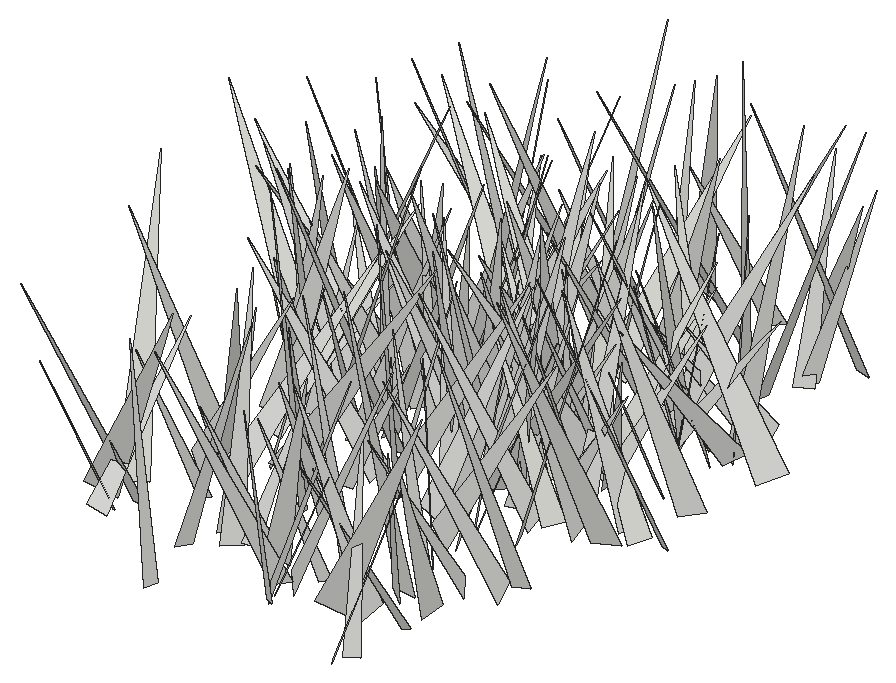
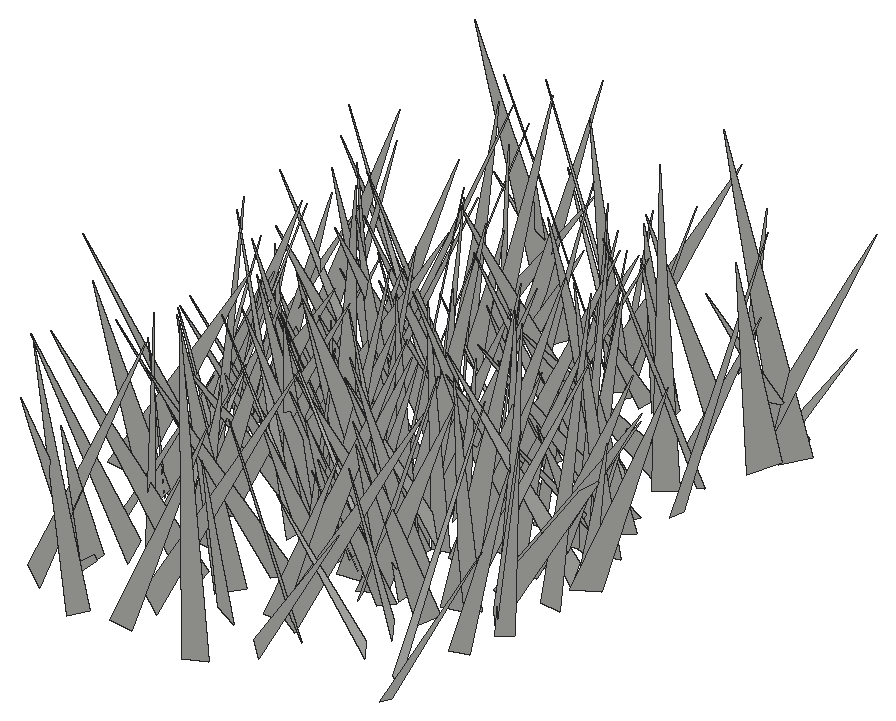
# SketchUp Ruby script. Lengths in inches.
U = 1.inch
M = Sketchup.active_model
def pt(a) = Geom::Point3d.new(a.map { |v| v * U })
def face(e, loops, mat)
  f = e.add_face(loops[0].map { |a| pt(a) })
  loops[1..].each { |l| e.add_face(l.map { |a| pt(a) }).erase! }
  f.material = f.back_material = mat if mat
  f
end
# faces: each face lists its corners as indices into pts; further lists are holes
def faces(e, pts, list, mat = nil) = list.each { |f| face(e, (f[0].is_a?(Array) ? f : [f]).map { |l| l.map { |i| pts[i] } }, mat) }
# xy, xz, yz: faces in a plane at the given z, y or x. An outline is a flat list of corners, or four numbers for a rectangle; further outlines are holes
def ring(l) = l.size == 4 ? [[l[0], l[1]], [l[2], l[1]], [l[2], l[3]], [l[0], l[3]]] : l.each_slice(2).to_a
def flat(e, list, mat, &to3) = list.each { |f| face(e, (f[0].is_a?(Array) ? f : [f]).map { |l| ring(l).map { |u, v| to3.(u, v) } }, mat) }
def xy(e, z, list, mat = nil) = flat(e, list, mat) { |x, y| [x, y, z] }
def xz(e, y, list, mat = nil) = flat(e, list, mat) { |x, z| [x, y, z] }
def yz(e, x, list, mat = nil) = flat(e, list, mat) { |y, z| [x, y, z] }
def lines(e, pts, list) = list.each { |a, b| e.add_line(pt(pts[a]), pt(pts[b])) }
# prism: a flat outline (further loops are holes) pulled along v
def prism(e, loops, v, mat = nil)
  f = face(e, loops, mat); d = Geom::Vector3d.new(v.map { |x| x * U })
  f.pushpull(f.normal.samedirection?(d) ? d.length : -d.length)
end
def box(e, o, s, mat = nil) = prism(e, [[o, [o[0] + s[0], o[1], o[2]], [o[0] + s[0], o[1] + s[1], o[2]], [o[0], o[1] + s[1], o[2]]]], [0, 0, s[2]], mat)
def at(x, y, z, deg = 0) = Geom::Transformation.translation(pt([x, y, z])) * Geom::Transformation.rotation(ORIGIN, Z_AXIS, deg.degrees)
def axes(o, x, y, z) = Geom::Transformation.new([*x, 0, *y, 0, *z, 0, *pt(o).to_a, 1])
def part(name) = M.definitions.add(name)
# library, detail: a bought-in or finely detailed component or shape, given as its bounding box
def library(name, o, s) = part(name).tap { |d| box(d.entities, o, s) }
def detail(e, o, s) = box(e.add_group.entities, o, s)
def put(e, d, t, mat = nil) = e.add_instance(d, t).tap { |i| i.material = mat if mat }
def group(e, t, mat = nil) = e.add_group.tap { |g| g.transformation = t; g.material = mat if mat }.entities
root = M.entities
c1 = part("fur_instance\#9")
p = [[0.8125,0,1.79],[0.67,-0.02,1.48],[0,-0.11,0],[0,0.11,0]]
faces(c1.entities,p,[[0,1,2,3]])
put(root,c1,axes([454.45,190.55,-21.66],[-5.80896,4.38047,0.69826],[4.41604,5.60261,1.59041],[-0.41794,-1.68592,7.09952]))
put(root,c1,axes([455.25,204.84,-21.66],[-4.70731,-0.314,0.0439],[-0.28456,4.4722,1.47573],[0.13983,-1.46975,4.48103]))
put(root,c1,axes([455.15,189.58,-21.66],[0.45308,4.94253,1.25959],[4.74966,-0.86975,1.70432],[-1.859,-1.01755,4.66145]))
put(root,c1,axes([455.2,175.94,-21.66],[-6.50457,4.89284,0.5628],[4.72218,6.46057,-1.59001],[1.39918,0.94188,7.98255]))
put(root,c1,axes([456.21,173.26,-21.66],[-2.80536,-2.90649,0.0794],[-2.63209,2.49174,-1.78533],[-1.23535,1.29136,3.62358]))
put(root,c1,axes([457.82,191.1875,-21.66],[-5.05806,4.73106,0.08976],[4.36112,4.60989,2.7757],[-1.83619,-2.08349,6.34527]))
put(root,c1,axes([456.97,193.71,-21.66],[-0.73144,-5.99959,0.26703],[-5.39662,0.53861,-2.681],[-2.63493,0.56233,5.41685]))
put(root,c1,axes([456.87,174.45,-21.66],[-2.83632,-6.0499,0.28173],[-5.90232,2.69141,-1.62612],[-1.35766,0.93829,6.48088]))
put(root,c1,axes([456.02,195.5,-21.66],[-4.69579,-3.74143,2.09942],[-4.25802,4.44495,-1.60248],[0.52452,2.58851,5.78625]))
put(root,c1,axes([455.65,182.05,-21.66],[-7.05336,-2.15617,1.71578],[-1.62887,7.06566,2.18314],[2.22256,-1.66441,7.04506]))
put(root,c1,axes([457.25,190.05,-21.66],[-3.27496,5.22829,1.96451],[5.47571,2.5569,2.32348],[-1.10043,-2.83671,5.71505]))
put(root,c1,axes([455.375,199.04,-21.66],[3.46395,-3.11936,0.86631],[-2.7787,-3.51575,-1.54862],[-1.66124,-0.62369,4.39672]))
put(root,c1,axes([454.77,192.86,-21.66],[-2.27672,-7.40144,1.23154],[-7.29478,2.48469,1.44709],[1.75622,0.72557,7.60728]))
put(root,c1,axes([456.03,203.05,-21.66],[-4.76858,-5.56642,0.65425],[-5.40433,4.79429,1.40014],[1.48534,-0.42682,7.19472]))
put(root,c1,axes([459.25,193.09,-21.66],[-5.59942,-5.49473,0.70955],[-5.42162,5.22657,-2.3104],[-1.14084,2.13071,7.49717]))
put(root,c1,axes([455.63,172.7,-21.66],[-0.63862,5.35473,0.03552],[5.1577,0.62471,-1.44573],[1.43964,0.13724,5.19527]))
put(root,c1,axes([458.1,185.21,-21.66],[-3.16034,-1.96863,0.75138],[-2.10046,2.8354,-1.40585],[-0.16774,1.5852,3.44773]))
put(root,c1,axes([454.72,196.38,-21.66],[-1.50636,-7.45489,0.25307],[-6.77182,1.47502,3.14252],[3.12761,-0.39686,6.92598]))
put(root,c1,axes([455.55,187.31,-21.66],[-0.42435,-6.57592,2.54627],[-6.78158,1.0798,1.65847],[1.93298,2.34469,6.37748]))
put(root,c1,axes([457.88,186.42,-21.66],[-4.70225,1.57903,0.9136],[0.9953,4.33742,-2.37389],[1.52885,2.03289,4.35536]))
put(root,c1,axes([458.82,176.93,-21.66],[-0.44719,-4.16584,0.88919],[-4.01944,0.11666,-1.47491],[-1.41032,0.98845,3.92158]))
put(root,c1,axes([459.29,189.81,-21.66],[-1.35626,4.67986,0.4324],[4.48876,1.15652,1.56235],[-1.3925,-0.82998,4.61514]))
put(root,c1,axes([455.82,189.625,-21.66],[6.85876,3.23862,0.41321],[3.02392,-6.66397,2.03701],[-1.23097,1.67477,7.30628]))
put(root,c1,axes([457.08,187.68,-21.66],[-3.46246,-6.72611,1.90114],[-6.59046,3.84836,1.61233],[2.32826,0.89059,7.39118]))
put(root,c1,axes([457.16,187.43,-21.66],[4.65411,-4.15615,0.09318],[-4.0063,-4.52139,-1.56511],[-1.10988,-1.10744,6.04026]))
put(root,c1,axes([456.25,186.42,-21.66],[-0.23722,4.19444,0.05409],[3.55446,0.22976,-2.22834],[2.22756,0.08005,3.56147]))
put(root,c1,axes([454.51,174.41,-21.66],[3.10816,-7.62871,0.22312],[-7.12075,-2.81203,3.04879],[2.74626,1.34273,7.65263]))
put(root,c1,axes([461.44,190.13,-21.66],[0.20171,6.63601,2.13173],[6.14884,-1.17367,3.07178],[-3.28217,-1.79094,5.8857]))
put(root,c1,axes([456.18,187.3125,-21.66],[3.26284,4.45559,0.15103],[4.26787,-3.06768,-1.7017],[1.28856,-1.1217,5.25381]))
put(root,c1,axes([459.2,199.33,-21.66],[4.53649,3.63122,1.57008],[3.09166,-4.74451,2.04009],[-2.46831,0.73111,5.44092]))
put(root,c1,axes([456.54,185.21,-21.66],[0.11593,7.32982,3.76994],[7.80213,1.11829,-2.4142],[2.6581,-3.60212,6.9218]))
put(root,c1,axes([460.31,190.17,-21.66],[2.04194,-5.37013,1.21962],[-4.97283,-2.35693,-2.05211],[-2.36574,0.31918,5.36625]))
put(root,c1,axes([457.5,195.51,-21.66],[0.9975,-5.62203,0.93729],[-5.55991,-0.75041,1.41599],[1.25425,1.14473,5.53148]))
put(root,c1,axes([457.11,183.9375,-21.66],[-1.44675,6.62808,0.1342],[5.91861,1.35324,-3.03008],[2.98656,0.529,6.06986]))
put(root,c1,axes([462.35,197.03,-21.66],[-5.71185,4.45959,0.23835],[4.39877,5.55102,1.55146],[-0.77178,-1.36683,7.07857]))
put(root,c1,axes([459.51,181.11,-21.66],[3.36886,3.17868,0.5186],[2.75759,-3.23451,1.91201],[-1.66392,1.0752,4.2187]))
put(root,c1,axes([458.05,195.9,-21.66],[7.18044,-3.7228,0.21814],[-3.29243,-6.55088,-3.42221],[-1.75122,-2.94828,7.32847]))
put(root,c1,axes([460.53,192.27,-21.66],[0.98136,-7.62341,0.77855],[-7.49654,-1.11781,-1.49599],[-1.58884,0.56543,7.53933]))
put(root,c1,axes([456.37,179.33,-21.66],[3.98085,5.13777,1.04709],[4.9615,-3.26572,-2.83883],[1.69606,-2.50573,5.84679]))
put(root,c1,axes([462.77,197.01,-21.66],[-7.75285,-2.01113,0.68817],[-2.11722,7.53738,-1.82488],[0.1887,1.94117,7.79879]))
put(root,c1,axes([461.73,187.27,-21.66],[2.76553,6.92914,2.18566],[6.51494,-3.40021,2.53621],[-3.21647,-0.92942,7.01632]))
put(root,c1,axes([459.09,201.59,-21.66],[4.51704,3.2359,0.24642],[3.07452,-4.40221,1.45028],[-1.0388,1.04161,5.3639]))
put(root,c1,axes([457.54,180.54,-21.66],[7.63705,-2.12328,0.08153],[-2.0044,-7.29978,-2.35267],[-0.70524,-2.24596,7.56953]))
put(root,c1,axes([458.59,179.22,-21.66],[-3.50989,5.55769,0.51718],[4.45011,3.15505,-3.70364],[3.36927,1.62248,5.4305]))
put(root,c1,axes([458.46,197.51,-21.66],[4.54931,-2.96003,1.24819],[-3.21199,-4.22741,1.68171],[-0.05363,2.09362,5.16041]))
put(root,c1,axes([462.23,168.58,-21.66],[-5.98582,-0.44068,0.88109],[-0.67667,5.78235,-1.70504],[0.71598,1.78068,5.75475]))
put(root,c1,axes([463.15,204.84,-21.66],[-3.16767,-3.69393,0.44061],[-3.42422,2.66901,-2.24153],[-1.45395,1.76199,4.31912]))
put(root,c1,axes([463.41,186.07,-21.66],[-3.74944,-6.99723,1.04952],[-6.92154,3.38084,-2.18706],[-1.468,1.93125,7.63127]))
put(root,c1,axes([460.03,187.05,-21.66],[-1.799,-4.93024,0.4482],[-4.7112,1.85147,1.45641],[1.52075,-0.09654,5.04207]))
put(root,c1,axes([463.42,178.71,-21.66],[-7.24108,-2.76695,1.69952],[-3.23599,6.49389,-3.21487],[0.2698,3.62643,7.05364]))
put(root,c1,axes([463.7,201.8,-21.66],[-2.5504,-6.61055,0.06946],[-6.29815,2.40698,-2.17909],[-2.00934,0.84606,6.74207]))
put(root,c1,axes([460.77,194.97,-21.66],[7.1916,2.06862,2.54607],[1.20326,-7.37063,2.58975],[-3.05186,1.96861,7.0208]))
put(root,c1,axes([463.9,183.93,-21.66],[-7.08449,-0.21202,0.14595],[-0.16992,6.87165,1.73429],[0.19334,-1.72965,6.8722]))
put(root,c1,axes([461.72,174.9,-21.66],[4.93577,0.48548,2.66433],[-0.37318,-5.36398,1.66873],[-2.68236,1.63958,4.67042]))
put(root,c1,axes([461.125,185.51,-21.66],[-5.44791,2.04028,1.98238],[0.64646,5.0587,-3.42987],[2.77031,2.83181,4.69878]))
put(root,c1,axes([462.83,174.07,-21.66],[-6.34351,2.24327,1.15963],[1.89857,6.30395,-1.80908],[1.66506,1.35834,6.48071]))
put(root,c1,axes([461.02,172.59,-21.66],[5.70541,0.17051,1.69377],[-0.31532,-5.71566,1.63753],[-1.67287,1.65887,5.46803]))
put(root,c1,axes([462.67,195.15,-21.66],[-4.26385,3.34064,0.29483],[3.15748,4.15963,-1.468],[1.13011,0.98225,5.21395]))
put(root,c1,axes([463.83,188.33,-21.66],[-6.21207,0.31771,0.7174],[0.09871,5.99609,-1.80072],[0.77837,1.77522,5.95384]))
put(root,c1,axes([461.47,182.03,-21.66],[6.96857,3.90701,1.2479],[3.36407,-6.85211,2.66731],[-2.34628,1.77954,7.53068]))
put(root,c1,axes([464.39,189.52,-21.66],[-6.62778,2.24684,1.33683],[2.5489,6.36376,1.94128],[0.58185,-2.2841,6.72363]))
put(root,c1,axes([464.28,201.01,-21.66],[-0.7633,-7.78268,1.04828],[-7.63293,0.4877,-1.93706],[-1.84592,1.20152,7.57632]))
put(root,c1,axes([462.75,202.24,-21.66],[4.10406,6.33899,0.98584],[6.11766,-4.2195,1.66374],[-1.93105,0.10466,7.36601]))
put(root,c1,axes([460.75,196.53,-21.66],[6.83601,2.20523,1.02382],[2.40175,-6.59991,-1.82073],[-0.37792,-2.05437,6.94831]))
put(root,c1,axes([462.09,180.84,-21.66],[5.97611,0.87511,2.00016],[1.66713,-5.59279,-2.53411],[-1.40966,-2.90435,5.48252]))
put(root,c1,axes([462.76,191.13,-21.66],[5.4592,3.52611,0.65952],[3.05756,-5.20187,2.50265],[-1.87611,1.78282,5.99776]))
put(root,c1,axes([462.05,187.125,-21.66],[6.79493,0.95964,1.40947],[0.56386,-6.72962,1.86359],[-1.60922,1.6941,6.60447]))
put(root,c1,axes([460.98,197.55,-21.66],[0.71966,5.69009,1.64056],[5.43341,0.02279,-2.46251],[2.35511,-1.79132,5.17987]))
put(root,c1,axes([464.45,201.9,-21.66],[1.33499,-4.14938,1.03511],[-3.92508,-1.61935,-1.42916],[-1.69781,0.48101,4.1179]))
put(root,c1,axes([462.26,191.83,-21.66],[-0.76172,-5.93829,1.58025],[-5.83151,1.20063,1.7008],[1.93753,1.27903,5.74028]))
put(root,c1,axes([463.48,174.57,-21.66],[-2.96386,2.60362,0.59977],[2.15648,2.85999,-1.75873],[1.5774,0.98217,3.53132]))
put(root,c1,axes([466.95,194.54,-21.66],[-5.54363,5.04114,0.10568],[4.92423,5.3789,1.72499],[-1.08457,-1.34553,7.29173]))
put(root,c1,axes([465.28,189.49,-21.66],[1.50286,-5.49819,1.33251],[-5.18917,-1.88889,-1.94134],[-2.25347,0.68284,5.35909]))
put(root,c1,axes([466.13,182.54,-21.66],[-6.09623,-2.24198,1.5344],[-2.70516,5.35755,-2.91953],[0.25098,3.28863,5.80232]))
put(root,c1,axes([464.22,195.45,-21.66],[-4.08665,1.67614,0.95166],[1.15635,3.91687,-1.93308],[1.54207,1.50482,3.97156]))
put(root,c1,axes([463.8,192.24,-21.66],[5.79186,-5.56058,1.06137],[-5.14067,-5.80215,-2.34538],[-2.37068,-1.00358,7.67886]))
put(root,c1,axes([464.62,174.78,-21.66],[-4.80536,-1.45342,1.08645],[-0.98448,4.67157,1.89512],[1.52434,-1.5647,4.64891]))
put(root,c1,axes([460.18,181.4,-21.66],[5.69226,-5.26322,0.96159],[-5.00885,-4.7486,3.65927],[1.88086,3.28288,6.8347]))
put(root,c1,axes([467.01,172.63,-21.66],[-0.65869,-6.64833,1.3688],[-6.16249,0.00919,-2.92087],[-2.84565,1.51902,6.00855]))
put(root,c1,axes([464.09,196.64,-21.66],[4.06405,-3.6671,0.18626],[-3.28339,-3.75381,-2.26428],[-1.64366,-1.56845,4.98369]))
put(root,c1,axes([464.62,195.49,-21.66],[2.09645,3.63188,0.13416],[3.39461,-2.01213,1.42535],[-1.29816,0.60366,3.94386]))
put(root,c1,axes([465.27,195.05,-21.66],[-4.827,3.94667,0.05385],[3.76525,4.62978,-1.80751],[1.18405,1.36675,5.96733]))
put(root,c1,axes([462.75,192.74,-21.66],[4.25693,-2.37845,0.80532],[-2.50825,-3.95225,1.586],[0.11926,1.77474,4.61119]))
put(root,c1,axes([464.63,179.14,-21.66],[4.72297,-1.05883,1.70864],[-0.28791,-4.67444,-2.10088],[-1.98939,-1.83725,4.36049]))
put(root,c1,axes([463.29,193.02,-21.66],[0.26156,-6.27199,1.2943],[-6.21893,0.06053,1.55008],[1.52905,1.31908,6.08306]))
put(root,c1,axes([463.37,181.89,-21.66],[3.09859,-2.8989,0.71648],[-2.92503,-2.73871,1.56906],[0.60101,1.61681,3.94246]))
put(root,c1,axes([466.35,203.15,-21.66],[1.43264,6.02249,0.66756],[5.77311,-1.565,1.72927],[-1.84042,-0.22107,5.94411]))
put(root,c1,axes([462.39,194.02,-21.66],[3.74419,-3.98525,0.35569],[-3.51637,-3.04515,2.89653],[1.90889,2.20738,4.63803]))
put(root,c1,axes([467.35,185.13,-21.66],[0.02975,6.47261,1.15989],[6.34372,-0.33363,1.69906],[-1.73125,-1.11127,6.2457]))
put(root,c1,axes([465.97,196.12,-21.66],[6.61822,-2.56323,1.80089],[-1.74555,-6.51281,-2.85492],[-2.60123,-2.15113,6.49773]))
put(root,c1,axes([467.625,170.89,-21.66],[1.94279,3.86541,2.10519],[3.74501,-2.66073,1.42935],[-2.3126,-1.06149,4.08323]))
put(root,c1,axes([462.99,195.6,-21.66],[5.8637,3.4963,0.04079],[3.31459,-5.53283,-2.23832],[1.11324,-1.94227,6.44958]))
put(root,c1,axes([468.4375,174.16,-21.66],[-1.09532,-3.977,1.33167],[-3.82769,0.38536,-1.99748],[-1.71426,1.68065,3.6092]))
put(root,c1,axes([466.73,195.8,-21.66],[-5.00496,1.9066,1.35129],[1.19771,4.83542,-2.3864],[2.00664,1.8693,4.79477]))
put(root,c1,axes([466.52,181.29,-21.66],[3.68113,4.53912,0.36663],[4.24955,-3.59341,1.82137],[-1.63686,0.87892,5.5531]))
put(root,c1,axes([469.94,204.42,-21.66],[-3.80092,-6.72254,0.0507],[-6.48684,3.65215,-2.05545],[-1.76524,1.05421,7.4441]))
put(root,c1,axes([464.75,207.48,-21.66],[-0.13317,-8.12567,1.45261],[-7.87911,0.55826,2.40046],[2.46092,1.34765,7.76415]))
put(root,c1,axes([466.48,187.2,-21.66],[6.75782,0.35235,2.65885],[1.16075,-6.88187,-2.03823],[-2.41791,-2.31896,6.45275]))
put(root,c1,axes([465.28,174.44,-21.66],[0.87943,-6.58228,1.27772],[-6.45662,-0.48373,1.95201],[1.80858,1.47376,6.34739]))
put(root,c1,axes([467.72,188.1,-21.66],[-6.44031,-4.10602,1.97316],[-3.85542,6.73281,1.42663],[2.42663,-0.20036,7.50344]))
put(root,c1,axes([469.95,174.32,-21.66],[-7.13799,-1.18277,0.6594],[-1.323,6.84565,-2.04241],[0.28881,2.12669,6.94107]))
put(root,c1,axes([467.82,189.51,-21.66],[-7.05102,3.6652,1.50452],[2.87345,6.84526,-3.20935],[2.72774,2.26338,7.26985]))
put(root,c1,axes([467.38,195.17,-21.66],[5.51307,6.12337,0.96272],[5.81555,-5.55551,2.03274],[-2.14519,0.67601,7.98483]))
put(root,c1,axes([467.47,195.44,-21.66],[-4.01189,-2.17426,1.82805],[-1.57492,4.33524,1.69992],[2.36407,-0.80168,4.23473]))
put(root,c1,axes([467.43,191.07,-21.66],[6.21031,-0.46369,2.15458],[0.49806,-5.98034,-2.72263],[-2.14689,-2.7287,5.60092]))
put(root,c1,axes([466.51,198.45,-21.66],[-0.73588,7.38124,0.25307],[6.98236,0.77818,-2.39362],[2.40696,-0.00075,7.02103]))
put(root,c1,axes([467.32,191.22,-21.66],[5.50822,-3.47682,2.75588],[-4.25576,-5.38219,1.71589],[-1.25366,2.99458,6.28367]))
put(root,c1,axes([470.95,189.15,-21.66],[-3.6214,4.75768,0.36392],[4.63089,3.39426,1.70771],[-1.15013,-1.31374,5.73008]))
put(root,c1,axes([468.86,185.6,-21.66],[-4.41847,1.33903,1.10997],[0.76139,4.21375,-2.05244],[1.56375,1.73183,4.13562]))
put(root,c1,axes([469.65,207.03,-21.66],[1.26749,-5.25605,0.55346],[-5.00773,-1.37633,-1.60227],[-1.68968,0.13629,5.16385]))
put(root,c1,axes([467.13,188.89,-21.66],[2.95876,-6.29379,1.88961],[-6.54545,-2.63888,1.45948],[0.58268,2.31543,6.79971]))
put(root,c1,axes([464.87,184.7,-21.66],[4.40787,6.56573,1.54887],[6.23945,-3.26461,-3.91775],[2.5646,-3.34225,6.86945]))
put(root,c1,axes([467.67,193.53,-21.66],[6.41211,-0.61612,1.30158],[-0.93497,-6.2989,1.62436],[-1.09524,1.77006,6.23347]))
put(root,c1,axes([470.96,191.92,-21.66],[-6.61706,2.95045,0.41304],[2.75432,6.44194,-1.89112],[1.13554,1.56763,6.99387]))
put(root,c1,axes([467.14,172.22,-21.66],[4.68379,1.41709,0.13919],[1.37897,-4.39495,-1.65779],[0.35492,-1.62533,4.60411]))
put(root,c1,axes([468.71,183.43,-21.66],[7.42059,-0.17453,3.00871],[-1.57677,-7.03899,3.48057],[-2.56838,3.81708,6.55601]))
put(root,c1,axes([467.47,194.25,-21.66],[2.98572,-5.88102,1.99527],[-6.13329,-2.44486,1.97166],[0.97482,2.63026,6.29392]))
put(root,c1,axes([467.12,171.55,-21.66],[6.01088,3.96881,0.98389],[4.08835,-5.80352,-1.56674],[0.06989,-1.84874,7.03046]))
put(root,c1,axes([468.05,192.33,-21.66],[0.34985,-8.1007,0.677],[-7.9597,-0.20383,1.67442],[1.6501,0.73429,7.93347]))
put(root,c1,axes([467.65,201.16,-21.66],[4.01839,-5.64573,1.18023],[-5.73753,-3.76564,1.52164],[0.58986,1.83314,6.76065]))
put(root,c1,axes([472.6,190.35,-21.66],[1.75618,-7.20882,1.45322],[-6.25973,-2.24953,-3.59425],[-3.85938,0.3683,6.49097]))
put(root,c1,axes([471.7,173.64,-21.66],[-2.56697,2.61634,0.35758],[2.51502,2.27032,1.44317],[-0.80484,-1.25014,3.36925]))
put(root,c1,axes([472.375,176.82,-21.66],[0.67019,6.07953,1.22269],[5.42193,-1.17133,2.85227],[-3.0097,-0.75637,5.41058]))
put(root,c1,axes([468.27,182.34,-21.66],[1.11802,6.55656,0.88639],[6.4324,-0.86675,-1.70208],[1.54866,-1.13332,6.42972]))
put(root,c1,axes([471.95,198.41,-21.66],[-1.56415,5.71782,0.81541],[5.62888,1.31989,1.54221],[-1.29382,-1.17019,5.72377]))
put(root,c1,axes([471.7,178.29,-21.66],[-4.19914,-2.372,1.71601],[-2.90919,3.71707,-1.98087],[0.32817,2.60017,4.39719]))
put(root,c1,axes([471.47,188.84,-21.66],[-5.20455,-0.25594,1.25726],[-0.61037,5.11409,-1.48563],[1.12857,1.58561,4.99457]))
put(root,c1,axes([472.22,175.56,-21.66],[1.71463,6.79892,3.94816],[7.36353,-2.80488,1.63226],[-2.7553,-3.26505,6.81916]))
put(root,c1,axes([467.35,173.01,-21.66],[5.84897,4.9177,0.90335],[4.92852,-5.43629,-2.31659],[0.84231,-2.33947,7.282]))
put(root,c1,axes([473.01,194.82,-21.66],[-1.63485,-6.2778,0.46595],[-5.97391,1.39539,-2.16005],[-1.98499,0.97094,6.117]))
put(root,c1,axes([472.77,184.83,-21.66],[-6.88482,-1.0416,0.48285],[-0.90858,6.73783,1.57954],[0.70182,-1.49517,6.78165]))
put(root,c1,axes([471.2,182.07,-21.66],[4.43621,4.25023,1.48293],[3.65379,-4.61591,2.29927],[-2.62932,0.75659,5.69717]))
put(root,c1,axes([471.03,185.28,-21.66],[-4.89219,1.92037,1.37183],[1.09822,4.64707,-2.5888],[2.08893,2.05431,4.57377]))
put(root,c1,axes([468.78,186.83,-21.66],[1.45839,-7.20301,2.88114],[-7.56056,-0.66269,2.17028],[1.73849,3.16049,7.02141]))
put(root,c1,axes([472.16,173.09,-21.66],[-6.75805,0.02177,1.99006],[0.56326,6.77748,1.83863],[1.90881,-1.92284,6.50317]))
put(root,c1,axes([472.52,201.22,-21.66],[-7.45834,-2.27512,2.73301],[-2.96816,7.48025,-1.87304],[1.95846,2.67246,7.56933]))
put(root,c1,axes([468.86,190.01,-21.66],[3.3459,3.39415,0.39754],[3.18536,-2.89609,-2.08314],[1.23764,-1.72213,4.2867]))
put(root,c1,axes([469.3,182.46,-21.66],[1.72384,-3.5656,0.8716],[-3.29525,-1.07913,2.10276],[1.61693,1.60212,3.35612]))
put(root,c1,axes([468.66,195.19,-21.66],[7.66511,2.45698,1.17946],[2.70747,-7.26796,-2.45522],[-0.3122,-2.70587,7.66567]))
put(root,c1,axes([473.59,185.17,-21.66],[-3.5373,3.73043,1.14853],[3.88761,3.22863,1.48666],[-0.34887,-1.84596,4.92122]))
put(root,c1,axes([474.41,172.89,-21.66],[-2.08934,-4.39389,0.06996],[-3.98317,1.86084,-2.08523],[-1.85622,0.95264,4.39584]))
put(root,c1,axes([469.09,186.125,-21.66],[6.564,-1.73993,0.0582],[-1.67851,-6.26496,2.01239],[0.46191,1.95953,6.48565]))
put(root,c1,axes([471.41,181.77,-21.66],[4.34106,2.99141,0.28027],[2.79242,-4.19877,1.56351],[-1.10882,1.13738,5.03476]))
put(root,c1,axes([469.33,201.51,-21.66],[7.73901,0.54751,0.09462],[0.50511,-7.48314,1.98706],[-0.23147,1.9758,7.49957]))
put(root,c1,axes([472.83,196.55,-21.66],[2.63198,-5.20128,0.6124],[-4.94839,-2.69423,-1.6156],[-1.71515,-0.20845,5.60093]))
put(root,c1,axes([474.2,189.4,-21.66],[-1.75901,-5.06572,0.78099],[-4.97011,1.48393,-1.5689],[-1.25276,1.22556,5.12778]))
put(root,c1,axes([470.58,186.23,-21.66],[4.65665,4.64477,2.8893],[5.46904,-4.02795,-2.33914],[-0.10763,-3.71592,6.14709]))
put(root,c1,axes([474.11,169.0625,-21.66],[0.39127,5.5531,0.09038],[5.24022,-0.39914,1.8382],[-1.83989,0.04412,5.25462]))
put(root,c1,axes([472,175.12,-21.66],[-2.28168,-4.43341,1.38047],[-4.1851,2.6298,1.52839],[2.0114,0.44265,4.74608]))
put(root,c1,axes([475.43,186.21,-21.66],[-3.98273,-4.40716,0.90523],[-4.3967,3.55588,-2.0321],[-0.95477,2.0093,5.58174]))
put(root,c1,axes([471.61,191.84,-21.66],[-2.11402,4.56513,0.60738],[3.84978,2.11854,-2.52378],[2.52756,0.59144,4.35202]))
put(root,c1,axes([473.9375,186.88,-21.66],[1.42623,8.08681,0.06748],[7.92603,-1.41139,1.61901],[-1.60595,0.21606,8.05043]))
put(root,c1,axes([474.0625,196.36,-21.66],[-5.99255,-5.60768,0.41861],[-5.37957,5.89507,1.95969],[1.63755,-1.155,7.96972]))
put(root,c1,axes([475.91,205.89,-21.66],[-4.08084,-6.31933,0.93728],[-6.28934,3.77891,-1.90517],[-1.12095,1.80323,7.27719]))
put(root,c1,axes([471.79,191.43,-21.66],[1.01067,5.88602,0.15693],[5.68933,-0.93518,-1.56469],[1.51703,-0.41415,5.76354]))
put(root,c1,axes([474.54,203.06,-21.66],[-5.37291,2.30629,0.61766],[1.96946,5.14098,-2.06404],[1.34972,1.6793,5.47055]))
put(root,c1,axes([474.01,177.8,-21.66],[-4.88167,-3.98465,0.29136],[-3.56929,4.55624,2.50876],[1.79514,-1.77658,5.7805]))
put(root,c1,axes([470.89,181.3,-21.66],[7.00496,3.81978,0.96353],[3.93839,-6.83549,-1.53416],[-0.09034,-1.80938,7.82984]))
put(root,c1,axes([474.51,198.42,-21.66],[-4.21387,-1.59887,0.24339],[-1.27519,3.70248,2.24451],[0.99474,-2.02671,3.90836]))
put(root,c1,axes([470.08,180.77,-21.66],[3.77376,6.10396,1.49671],[5.76595,-2.66802,-3.65722],[2.50047,-3.05991,6.17449]))
put(root,c1,axes([473.72,194.54,-21.66],[-3.75985,-4.2409,1.14983],[-3.97997,3.92819,1.47409],[1.86202,-0.16705,5.47255]))
put(root,c1,axes([473.3125,195.58,-21.66],[-6.68782,-2.79113,3.18251],[-2.04813,7.34131,2.13449],[3.70459,-0.98003,6.92541]))
put(root,c1,axes([474.93,185.52,-21.66],[-7.14717,-1.7401,1.8273],[-1.33254,7.26397,1.70532],[2.14274,-1.28679,7.15555]))
put(root,c1,axes([473.65,168.16,-21.66],[3.6245,2.89722,0.22495],[2.66528,-3.45765,1.58821],[-1.15791,1.11007,4.35987]))
put(root,c1,axes([470.43,172.1875,-21.66],[3.82613,-7.13137,0.63835],[-6.75778,-3.35774,2.99351],[2.36564,1.94225,7.51895]))
put(root,c1,axes([473.24,182.89,-21.66],[6.6915,4.26773,1.20587],[3.94044,-6.72308,1.92792],[-2.03484,1.01512,7.69888]))
put(root,c1,axes([476.1875,179.44,-21.66],[-1.63613,-6.00923,1.56488],[-6.02721,1.14742,-1.89548],[-1.49415,1.95172,5.93253]))
put(root,c1,axes([475.85,178.53,-21.66],[-6.75502,-2.37628,0.59319],[-2.11002,6.52988,2.13012],[1.24354,-1.82836,6.83664]))
put(root,c1,axes([477.8,186.45,-21.66],[-2.08516,6.03207,0.25096],[5.29839,1.7011,3.1353],[-2.89412,-1.23172,5.5591]))
put(root,c1,axes([472.33,186.97,-21.66],[1.50617,-3.93782,1.16858],[-3.70084,-0.76096,2.20573],[1.78207,1.74788,3.59301]))
put(root,c1,axes([472.62,186.74,-21.66],[1.91277,-3.82749,0.78831],[-3.61325,-1.39793,1.9799],[1.48846,1.5251,3.7932]))
put(root,c1,axes([475.08,192.35,-21.66],[4.44395,3.96646,1.43413],[3.47391,-4.62357,2.02305],[-2.39195,0.65422,5.60257]))
put(root,c1,axes([473.61,201.11,-21.66],[6.82922,2.21825,1.16198],[1.82522,-6.72015,2.10172],[-1.71447,1.68168,6.86597]))
put(root,c1,axes([475.22,194.88,-21.66],[-4.26482,-5.03014,0.77761],[-4.82923,4.31941,1.45497],[1.60794,-0.36894,6.43227]))
put(root,c1,axes([473.22,190.01,-21.66],[5.22724,-1.35677,0.09683],[-1.28473,-5.05093,-1.4184],[-0.44684,-1.34966,5.21086]))
put(root,c1,axes([472,207.37,-21.66],[1.01842,-6.5564,0.3467],[-5.92672,-0.76709,2.90332],[2.82498,0.75429,5.9661]))
put(root,c1,axes([476.19,198.77,-21.66],[-4.14982,-0.72477,0.23143],[-0.53834,3.70403,1.94686],[0.53763,-1.88541,3.73578]))
put(root,c1,axes([478.96,195.16,-21.66],[-4.49913,6.58347,1.21187],[6.27218,3.63575,3.53468],[-2.33889,-2.91414,7.14775]))
put(root,c1,axes([474.39,174.91,-21.66],[5.34642,-2.10558,1.0321],[-1.67954,-5.23165,-1.97278],[-1.63641,-1.50973,5.39684]))
put(root,c1,axes([473.07,189.75,-21.66],[2.06268,4.77096,0.10661],[4.57909,-1.94603,-1.50762],[1.34363,-0.69206,4.97431]))
put(root,c1,axes([472.15,195.4,-21.66],[2.96543,7.80813,0.73471],[7.53088,-2.61577,-2.59693],[2.18919,-1.57838,7.9383]))
put(root,c1,axes([476.51,195.17,-21.66],[3.82585,4.29132,1.89582],[3.55577,-4.24822,2.44044],[-3.06039,0.42878,5.20545]))
put(root,c1,axes([476.65,187.34,-21.66],[-6.00437,2.1113,1.91932],[2.55574,5.96789,1.43049],[1.26869,-2.0299,6.20191]))
put(root,c1,axes([474.47,203.61,-21.66],[4.97283,-0.90694,1.68915],[-1.45035,-4.85051,1.66547],[-1.25389,2.01364,4.77261]))
put(root,c1,axes([475.8,196.56,-21.66],[7.23662,0.86237,3.59764],[-0.54989,-7.56504,2.91946],[-3.65846,2.84288,6.67751]))
put(root,c1,axes([476.71,185.3,-21.66],[0.82289,-7.98079,0.80674],[-7.83354,-0.97405,-1.64552],[-1.72608,0.61581,7.85254]))
put(root,c1,axes([479.12,186.74,-21.66],[-4.75874,-5.64309,0.42264],[-5.39038,4.3522,-2.58279],[-1.72245,1.97043,6.91515]))
put(root,c1,axes([476.39,195.56,-21.66],[3.78174,-4.82109,0.17581],[-4.12071,-3.34423,-3.06777],[-2.50869,-1.77444,5.30408]))
put(root,c1,axes([475.41,190.95,-21.66],[-2.3415,-4.6423,0.1365],[-4.37976,2.25803,1.66471],[1.54509,-0.63449,4.92568]))
put(root,c1,axes([478.11,190.1,-21.66],[1.0703,-6.74535,2.51722],[-6.58595,-1.94546,-2.41292],[-2.90886,1.9228,6.3893]))
put(root,c1,axes([473.07,194.68,-21.66],[3.04424,4.32162,0.01521],[3.85535,-2.70735,-2.39804],[1.95268,-1.39208,4.71097]))
